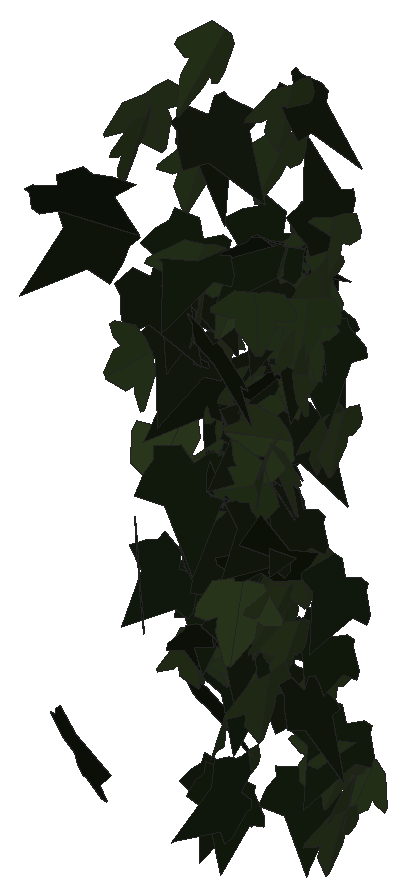
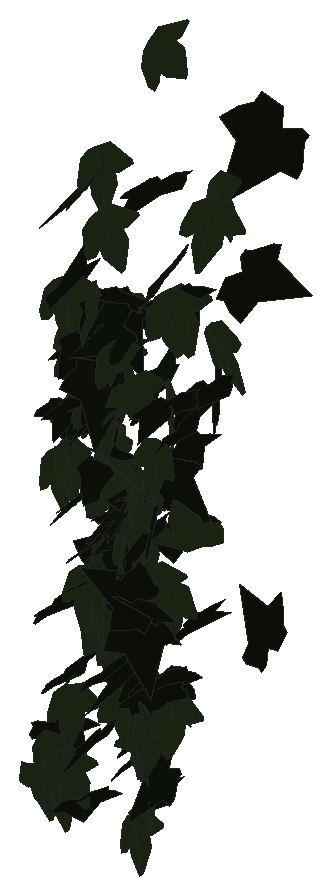
# SketchUp Ruby script. Lengths in inches.
U = 1.inch
M = Sketchup.active_model
def pt(a) = Geom::Point3d.new(a.map { |v| v * U })
def face(e, loops, mat)
  f = e.add_face(loops[0].map { |a| pt(a) })
  loops[1..].each { |l| e.add_face(l.map { |a| pt(a) }).erase! }
  f.material = f.back_material = mat if mat
  f
end
# faces: each face lists its corners as indices into pts; further lists are holes
def faces(e, pts, list, mat = nil) = list.each { |f| face(e, (f[0].is_a?(Array) ? f : [f]).map { |l| l.map { |i| pts[i] } }, mat) }
# xy, xz, yz: faces in a plane at the given z, y or x. An outline is a flat list of corners, or four numbers for a rectangle; further outlines are holes
def ring(l) = l.size == 4 ? [[l[0], l[1]], [l[2], l[1]], [l[2], l[3]], [l[0], l[3]]] : l.each_slice(2).to_a
def flat(e, list, mat, &to3) = list.each { |f| face(e, (f[0].is_a?(Array) ? f : [f]).map { |l| ring(l).map { |u, v| to3.(u, v) } }, mat) }
def xy(e, z, list, mat = nil) = flat(e, list, mat) { |x, y| [x, y, z] }
def xz(e, y, list, mat = nil) = flat(e, list, mat) { |x, z| [x, y, z] }
def yz(e, x, list, mat = nil) = flat(e, list, mat) { |y, z| [x, y, z] }
def lines(e, pts, list) = list.each { |a, b| e.add_line(pt(pts[a]), pt(pts[b])) }
# prism: a flat outline (further loops are holes) pulled along v
def prism(e, loops, v, mat = nil)
  f = face(e, loops, mat); d = Geom::Vector3d.new(v.map { |x| x * U })
  f.pushpull(f.normal.samedirection?(d) ? d.length : -d.length)
end
def box(e, o, s, mat = nil) = prism(e, [[o, [o[0] + s[0], o[1], o[2]], [o[0] + s[0], o[1] + s[1], o[2]], [o[0], o[1] + s[1], o[2]]]], [0, 0, s[2]], mat)
def at(x, y, z, deg = 0) = Geom::Transformation.translation(pt([x, y, z])) * Geom::Transformation.rotation(ORIGIN, Z_AXIS, deg.degrees)
def axes(o, x, y, z) = Geom::Transformation.new([*x, 0, *y, 0, *z, 0, *pt(o).to_a, 1])
def part(name) = M.definitions.add(name)
# library, detail: a bought-in or finely detailed component or shape, given as its bounding box
def library(name, o, s) = part(name).tap { |d| box(d.entities, o, s) }
def detail(e, o, s) = box(e.add_group.entities, o, s)
def put(e, d, t, mat = nil) = e.add_instance(d, t).tap { |i| i.material = mat if mat }
def group(e, t, mat = nil) = e.add_group.tap { |g| g.transformation = t; g.material = mat if mat }.entities
root = M.entities
M.materials.add("efeu1").color = [18, 25, 13]
M.materials.add("efeu2").color = [43, 57, 29]
c1 = part("ivyleaf_10")
p = [[0,0.5,-0.03],[-0.0625,2.02,-0.43],[-0.19,2.01,-0.46],[-0.54,1.05,-0.29],[-0.52,0.625,-0.18],[-0.83,0.76,-0.28],
  [-1.16,0.64,-0.33],[-1.15,0.33,-0.24],[-0.77,-0.39,0.02],[-0.3,-0.51,0.16],[0.04,-0.48,0.23],[-0.02,2.01,-0.4375],
  [-0.06,2.01,-0.43],[0.04,-0.49,0.23],[0.67,-0.49,0.14],[1.38,0.36,-0.2],[1.375,0.51,-0.24],[0.81,0.65,-0.19],
  [0.62,0.59,-0.15],[0.6,1.09,-0.28],[0.5,1.23,-0.31]]
faces(c1.entities,p,[[0,1,2,3,4,5,6,7,8,9,10],[11,12,0,13,14,15,16,17,18,19,20]],"efeu2")
c2 = part("ivyleaf_9")
p = [[1.54,2.16,1.25],[1.36,2.04,1.19],[-0.21,0.99,0.68],[-0.71,1.11,0.82],[-0.85,0.86,0.67],[-0.8,0.17,0.21],
  [-0.9,-0.01,0.1],[-0.67,-0.16,-0.02],[-0.08,-0.08,-0.05],[-0.03,-0.6,-0.4],[0.65,-0.88,-0.66],[0.83,-0.6,-0.49],
  [1.29,-0.42,-0.43],[1.8125,-0.07,-0.26],[1.21,0.44,0.15]]
faces(c2.entities,p,[[0,1,2,3,4,5,6,7,8,9,10,11,12,13,14]],"efeu1")
put(root,c1,axes([530.12,130.77,247.7],[0.59949,0.80925,0.19453],[-0.00458,0.24295,-0.99653],[-0.83229,0.58156,0.14561]))
put(root,c1,axes([530.45,128.96,248.09],[-0.34257,-0.93883,-0.20194],[0.053,0.1956,-0.99924],[0.95884,-0.34624,-0.01692]))
put(root,c2,axes([530.03,129.84,245.78],[0.99528,-0.08963,-0.19402],[-0.19533,-0.00644,-0.99903],[0.08673,1.014,-0.0235]))
put(root,c2,axes([530.17,128.98,261.25],[-0.11198,-1.02799,0.34018],[-0.0593,-0.33566,-1.03385],[1.08119,-0.12488,-0.02147]))
put(root,c1,axes([530.56,128.79,253.32],[-1.05087,0.04613,0.0573],[-0.05724,0.00251,-1.05188],[-0.0462,-1.05242,0]))
put(root,c2,axes([530.78,123.8,266.09],[-0.11934,0.03025,-1.214],[0.21164,-1.20066,-0.05073],[-1.19579,-0.21552,0.11218]))
put(root,c2,axes([530.32,129.95,249.92],[-0.34985,-0.95472,-0.20152],[0.09174,0.18095,-1.01653],[0.97143,-0.36092,0.02343]))
put(root,c2,axes([530.16,130.55,249.63],[-0.1055,-0.93069,-0.43752],[0.16886,0.41817,-0.93025],[1.01444,-0.16639,0.10934]))
put(root,c2,axes([530.61,127.8,251.39],[-0.44294,-0.72773,0.60696],[-0.1684,-0.59888,-0.84094],[0.93254,-0.45381,0.13644]))
put(root,c1,axes([530.68,130.96,248.01],[0.15636,-0.97706,-0.24122],[-0.00188,0.24383,-0.98885],[1.00639,0.15226,0.03563]))
put(root,c2,axes([530.94,129.91,256.45],[0.03772,-0.47428,0.94553],[-0.09107,0.94116,0.47572],[-1.05389,-0.0983,-0.00727]))
put(root,c2,axes([530.18,127.08,262.39],[0.26239,-0.86938,-0.67513],[-0.04832,0.68428,-0.89994],[1.09967,0.23751,0.12155]))
put(root,c1,axes([530.3125,127.43,255.44],[1.01001,0.43056,-0.45145],[0.33211,0.35614,1.08267],[0.52811,-1.04742,0.18255]))
put(root,c1,axes([530.84,129.98,245.01],[0.35064,-0.78367,-0.54081],[-0.16794,0.51638,-0.85715],[0.93724,0.38571,0.04874]))
put(root,c1,axes([530.45,130.86,248.88],[0.85042,-0.50683,0.25032],[0.22614,-0.1094,-0.98977],[0.51807,0.87971,0.02113]))
put(root,c1,axes([530.82,129.52,260.12],[-1.0224,0.29815,0.06081],[-0.05654,0.02331,-1.06497],[-0.29899,-1.02394,-0.00654]))
put(root,c1,axes([530.89,128.79,266.59],[-0.35003,-1.00823,0.27449],[-0.0023,-0.28874,-1.06349],[1.04492,-0.33837,0.08961]))
put(root,c2,axes([531.1,130.24,252.35],[0.13928,0.95863,-0.39167],[-0.04693,-0.38895,-0.96866],[-1.0345,0.14671,-0.00879]))
put(root,c1,axes([530.89,125.92,269.74],[-0.5113,-1.01793,-0.36269],[0.15271,0.32915,-1.13908],[1.06977,-0.53351,-0.01075]))
put(root,c2,axes([530.77,128.34,259.86],[-0.42963,-0.9869,0.13227],[-0.03846,-0.12751,-1.07625],[0.99498,-0.43107,0.01552]))
put(root,c1,axes([530.85,129.02,248.5],[-0.89116,-0.4413,-0.29325],[0.28362,0.08738,-0.9934],[0.44755,-0.93409,0.04561]))
put(root,c1,axes([531.07,130.58,243.11],[-0.05678,-1.01777,-0.0273],[0.00058,0.02731,-1.01936],[1.01814,-0.05677,-0.00094]))
put(root,c2,axes([531.45,128.48,258.46],[0.05872,0.39433,-1.01387],[-0.24983,-0.98332,-0.39692],[-1.05878,0.25389,0.03743]))
put(root,c2,axes([531.35,128.67,249.0625],[0.34784,0.92965,-0.39975],[-0.14348,-0.37312,-0.99259],[-1.00173,0.37626,0.00337]))
put(root,c2,axes([530.73,128.94,262.32],[0.09413,-0.9504,-0.53101],[0.10933,0.53855,-0.94452],[1.08318,0.02823,0.14148]))
put(root,c2,axes([531.2,130.58,253.4],[-0.77358,-0.58488,-0.36776],[0.33791,0.16126,-0.96725],[0.60262,-0.84123,0.07027]))
put(root,c2,axes([530.97,129.97,256.48],[0.41315,-0.87903,-0.41991],[-0.20592,0.367,-0.97089],[0.95216,0.46079,-0.02777]))
put(root,c1,axes([531.28,129.68,257.39],[0.15332,1.02837,-0.21556],[-0.11788,-0.19963,-1.03623],[-1.04409,0.17355,0.08534]))
put(root,c2,axes([531.07,130.69,246.36],[-0.00824,-0.96592,0.32251],[0.05102,-0.32251,-0.96461],[1.01706,0.00835,0.051]))
put(root,c1,axes([531.6,127.72,261.8125],[0.5825,-0.86043,-0.34942],[-0.07373,0.36832,-1.02987],[0.92574,0.57074,0.13784]))
put(root,c2,axes([531.18,129.97,253.33],[0.30859,0.94921,-0.32028],[0.11588,0.29906,0.99797],[0.99506,-0.3292,-0.0169]))
put(root,c1,axes([531.76,124.38,269.77],[0.25662,-1.08207,0.21063],[0.06001,-0.20223,-1.11202],[1.10074,0.26329,0.01152]))
put(root,c1,axes([531.97,128.47,253.37],[-0.41024,-0.92186,0.25569],[-0.07056,-0.24829,-1.0084],[0.95406,-0.41476,0.03536]))
put(root,c2,axes([531.27,128.5,267.68],[0.37366,-1.0709,0.30288],[0.11181,-0.28175,-1.13415],[1.10728,0.38983,0.01232]))
put(root,c2,axes([531.57,127.48,255.68],[-0.32244,-1.11278,-0.29915],[0.12901,0.27382,-1.15764],[1.14505,-0.3442,0.04619]))
put(root,c1,axes([531.8,129.71,258.05],[0.27073,-0.96086,0.35696],[0.19498,-0.31419,-0.9936],[1.00631,0.31938,0.09648]))
put(root,c1,axes([532.11,129.26,255.74],[-0.54822,-0.8563,0.28432],[-0.05627,-0.29959,-1.0108],[0.90051,-0.54003,0.10992]))
put(root,c2,axes([531.93,129.22,251.79],[-0.84528,-0.4313,-0.44212],[0.3754,0.23632,-0.94827],[0.49047,-0.92419,-0.03615]))
put(root,c2,axes([531.79,128.94,243.3125],[-0.20911,-0.94123,0.33342],[-0.04181,-0.3321,-0.96372],[0.99766,-0.2112,0.02949]))
put(root,c1,axes([532.08,129.51,256.86],[0.19886,-1.04332,-0.15253],[0.06117,0.16638,-1.05826],[1.05264,0.18743,0.09031]))
put(root,c1,axes([532.67,123.26,262.1],[0.74777,-0.37964,-0.89561],[-0.74706,0.49937,-0.83542],[0.62301,1.05446,0.07319]))
put(root,c2,axes([531.34,121.66,247.56],[0.15407,-0.39236,1.1611],[0.65177,-0.96482,-0.41251],[1.03793,0.66409,0.08669]))
put(root,c2,axes([531.78,129.83,250.04],[0.47251,-0.61408,-0.7153],[-0.14645,0.74259,-0.73425],[0.93129,0.42834,0.24746]))
put(root,c1,axes([532.35,129.43,255.29],[0.13488,-1.05588,-0.0346],[0.00799,0.0359,-1.06439],[1.05642,0.13454,0.01247]))
put(root,c2,axes([533.11,129.66,258.89],[-0.73823,0.61644,0.46097],[-0.48636,0.12149,-0.94136],[-0.59661,-0.86181,0.19702]))
put(root,c1,axes([532.46,129.04,262.41],[0.53412,0.82489,-0.43726],[-0.3576,-0.28459,-0.97368],[-0.86242,0.62888,0.13292]))
put(root,c1,axes([532.625,129.3125,247.85],[-0.89132,-0.47812,0.19014],[-0.15564,-0.11197,-1.01116],[0.49044,-0.90447,0.02466]))
put(root,c2,axes([532.01,128.99,255.09],[0.38304,-0.99677,0.07006],[0.01635,-0.06877,-1.06779],[0.99909,0.38328,-0.00939]))
put(root,c2,axes([532.13,129.96,257.41],[0.79649,-0.69692,-0.08546],[-0.05915,0.06217,-1.05832],[0.69964,0.79865,0.00781]))
put(root,c1,axes([533,125.9375,264.74],[-0.54976,-0.95739,0.43782],[-0.16961,-0.40692,-1.1028],[1.03899,-0.57301,0.05164]))
put(root,c2,axes([532.94,127.5625,252.09],[-1.03158,0.08408,0.36527],[0.36419,-0.02808,1.035],[0.08863,1.09398,-0.0015]))
put(root,c1,axes([532.8,129.6875,258.23],[0.14132,0.795,-0.70096],[-0.23378,-0.66637,-0.8029],[-1.03379,0.25937,0.08575]))
put(root,c2,axes([532.47,129.91,256.16],[0.07819,-1.05398,0.07923],[0.00586,-0.07901,-1.05688],[1.05694,0.07841,0]))
put(root,c2,axes([532.11,130.0625,255.08],[0.49608,-0.63665,0.68073],[0.40886,-0.54435,-0.80705],[0.83759,0.64278,-0.00923]))
put(root,c2,axes([532.54,128.96,249.57],[-0.06401,-0.9947,0.27218],[0.06025,-0.27584,-0.99392],[1.0295,-0.0457,0.07509]))
put(root,c2,axes([532.56,129.82,256.64],[0.04567,-1.05775,0.09583],[-0.00293,-0.09605,-1.05871],[1.06208,0.04522,-0.00704]))
put(root,c2,axes([532.92,126.19,265.15],[-0.55878,-0.95758,0.09599],[-0.0309,-0.09309,-1.10851],[0.96188,-0.55927,0.02015]))
put(root,c2,axes([532.65,119.27,270.13],[1.09209,0.78995,0.16363],[0.13161,0.09724,-1.34784],[-0.79591,1.09999,0.00164]))
put(root,c2,axes([533.45,129.6,258.75],[-0.24559,0.82548,-0.63707],[-0.04422,-0.66216,-0.84094],[-1.04178,-0.16649,0.18587]))
put(root,c1,axes([533.04,129.45,261.01],[-0.18241,1.05483,0.06532],[-0.04393,0.05866,-1.06996],[-1.05593,-0.18466,0.03323]))
put(root,c2,axes([533.26,129.39,256.63],[-0.57729,-0.69178,0.56472],[-0.18522,-0.56507,-0.88155],[0.87359,-0.57695,0.18628]))
put(root,c2,axes([533.16,130.1,249.36],[-0.22242,-0.96615,0.28906],[0.04103,-0.30443,-0.98595],[1.00763,-0.20087,0.10396]))
put(root,c2,axes([533.01,130.55,246.76],[0.50348,-0.70739,-0.51884],[-0.12405,0.53479,-0.84952],[0.86845,0.4865,0.17944]))
put(root,c1,axes([533.35,129.61,258.51],[-0.8221,-0.61552,-0.30437],[0.31377,0.08559,-1.02058],[0.61078,-0.87245,0.11462]))
put(root,c2,axes([533.75,129.35,262.59],[0.2989,1.03665,-0.02085],[-0.16913,0.02734,-1.0654],[-1.02297,0.29838,0.17005]))
put(root,c1,axes([533.63,128.82,263.39],[-0.17447,-1.06916,0.16961],[-0.004,-0.17116,-1.08305],[1.08252,-0.17295,0.02333]))
put(root,c1,axes([534.35,127.41,256.11],[-0.46385,-0.03418,1.01927],[-0.99443,-0.23328,-0.46037],[0.22627,-1.09529,0.06625]))
put(root,c2,axes([533.33,129.21,255.11],[-0.02323,-1.05348,-0.00984],[0.00051,0.00983,-1.05373],[1.05352,-0.02323,0.00029]))
put(root,c1,axes([533.74,129.14,254.44],[-0.12558,-1.04555,-0.18309],[0.03647,0.18001,-1.05297],[1.06084,-0.12996,0.01453]))
put(root,c1,axes([533.625,127.24,251.7],[1.06375,0.44099,-0.03659],[-0.03726,-0.00567,-1.1515],[-0.44094,1.06436,0.00903]))
put(root,c1,axes([533.88,129.18,252.36],[0.12962,-1.02698,-0.23441],[0.03802,0.24058,-1.03301],[1.05271,0.11776,0.06617]))
put(root,c2,axes([533.04,126.74,261.02],[0.52164,-0.91056,0.61644],[0.37199,-0.49593,-1.04734],[1.03477,0.63731,0.06575]))
put(root,c1,axes([533.9375,128.62,261.89],[-0.87984,0.6414,0.04331],[-0.03262,0.02877,-1.0888],[-0.64203,-0.88044,-0.00403]))
put(root,c2,axes([533.73,126.8,244.75],[-0.11574,-1.00161,0.18712],[0.04156,-0.19281,-1.00635],[1.0181,-0.10599,0.06236]))
put(root,c1,axes([534.83,127.69,257.83],[0.27933,0.01691,-1.05814],[-1.02728,0.26726,-0.26691],[0.25426,1.06125,0.08408]))
put(root,c2,axes([534.64,127.64,264.93],[0.07292,0.8712,-0.65607],[-0.31199,-0.61339,-0.84921],[-1.04503,0.24392,0.20775]))
put(root,c1,axes([534.32,128.58,250.46],[0.01689,-1.05078,-0.14834],[-0.02901,0.14784,-1.05059],[1.06081,0.02077,-0.02636]))
put(root,c2,axes([533.67,125.77,270.21],[0.26945,-0.9044,-0.61716],[0.13905,0.65869,-0.90456],[1.08604,0.14005,0.26893]))
put(root,c2,axes([533.96,130.54,243.32],[-0.26686,-0.97619,-0.13817],[0.18499,0.09102,-1.00037],[0.9684,-0.28639,0.15302]))
put(root,c2,axes([534.71,128.9375,263.74],[0.17806,0.76682,-0.74846],[-0.36329,-0.67059,-0.77346],[-1.00808,0.37711,0.14654]))
put(root,c1,axes([534.78,130.59,244.76],[-0.79743,-0.30381,0.53872],[-0.45971,-0.29688,-0.8479],[0.41375,-0.9154,0.09619]))
put(root,c1,axes([534.48,128.35,251.48],[0.04459,-1.02604,0.41002],[-0.00398,-0.4105,-1.02681],[1.10492,0.03993,-0.02025]))
put(root,c2,axes([534.41,127.97,254.11],[-0.45426,-0.68394,0.65485],[-0.04892,-0.70839,-0.77379],[0.94562,-0.36519,0.27454]))
put(root,c2,axes([534.83,127.91,265.32],[-0.98302,-0.46707,0.08796],[-0.07577,-0.04549,-1.0883],[0.46921,-0.98589,0.00854]))
put(root,c2,axes([534.35,128.4375,262.99],[-0.35633,-1.0252,0.15593],[0.00596,-0.1669,-1.08371],[1.03697,-0.35132,0.05981]))
put(root,c2,axes([533.87,128.16,264.42],[1.02581,0.09267,0.36656],[0.34215,0.22356,-1.014],[-0.16091,1.06615,0.18076]))
put(root,c2,axes([534.01,129.53,261.43],[-0.38886,-0.2086,-0.97796],[0.84515,0.49227,-0.44105],[0.53445,-0.93021,-0.0141]))
put(root,c1,axes([534.72,130.34,247.7],[-0.33241,-0.96187,-0.10175],[0.02363,0.09949,-1.01764],[0.96695,-0.33309,-0.01011]))
put(root,c2,axes([534.26,129.6,260.5],[0.04716,-1.01184,0.34823],[0.01958,-0.34769,-1.01293],[1.0699,0.05096,0.00319]))
put(root,c2,axes([534.42,127.47,252.88],[0.94663,0.32897,0.50604],[-0.47408,-0.17731,1.0021],[0.37356,-1.05865,-0.01059]))
put(root,c1,axes([534.92,127.9375,268.7],[-0.29245,-0.99715,0.41347],[-0.09535,-0.40284,-1.03895],[1.07525,-0.30693,0.02033]))
put(root,c1,axes([534.98,129.07,263.01],[-1.00927,-0.36391,0.1748],[-0.14593,-0.11,-1.07155],[0.37642,-1.01837,0.05328]))
put(root,c1,axes([534.68,127.93,257.02],[-0.89144,0.54624,-0.16724],[0.15477,-0.06743,-1.04523],[-0.5499,-0.90448,-0.02308]))
put(root,c1,axes([534.91,129.06,252.66],[-0.34895,-0.97798,-0.17168],[0.02509,0.17324,-1.03781],[0.99262,-0.34818,-0.03413]))
put(root,c2,axes([534.29,129.66,257.32],[0.44249,-0.89305,-0.33876],[0.04898,0.39407,-0.97488],[0.95388,0.39404,0.2072]))
put(root,c2,axes([534.6,129.28,254.375],[-0.3017,-0.87595,0.49937],[0.07577,-0.53947,-0.90051],[1.00544,-0.22219,0.21771]))
put(root,c1,axes([534.88,128.5,250.21],[0.02965,-0.97597,0.35183],[0.10646,-0.34725,-0.97224],[1.03197,0.06386,0.09019]))
put(root,c1,axes([534.79,128.99,261.4375],[0.2457,1.05115,0.08164],[-0.09951,0.10658,-1.0727],[-1.04961,0.23596,0.12081]))
put(root,c1,axes([535.03,126.9,249.06],[-0.12949,-1.19814,-0.09629],[0.01443,0.09529,-1.20511],[1.20191,-0.13023,0.00409]))
put(root,c2,axes([534.71,130.69,249.02],[-0.21835,-0.93375,0.34678],[0.02703,-0.36044,-0.95351],[0.9957,-0.19498,0.10193]))
put(root,c1,axes([534.8,129.03,265.09],[-0.03865,0.37648,-1.02131],[0.09702,-1.0167,-0.37845],[-1.08416,-0.10441,0.00254]))
put(root,c2,axes([535.73,124.6,246.3],[-1.03988,0.40389,0.05562],[-0.0546,0.01304,-1.11554],[-0.40403,-1.04129,0.00761]))
put(root,c2,axes([534.74,129.79,261.39],[0.09441,-0.96076,-0.45432],[0.05777,0.46007,-0.96092],[1.06119,0.06043,0.09273]))
put(root,c1,axes([535.42,125.99,263.83],[-0.89328,-0.63308,0.04333],[-0.0364,-0.02357,-1.09487],[0.63351,-0.89402,-0.00181]))
put(root,c1,axes([534.9,127.18,257.3],[-0.17418,-0.2576,-1.08193],[0.30362,-1.06454,0.20458],[-1.06993,-0.26015,0.23419]))
put(root,c2,axes([535.17,129.66,260.98],[-0.42013,-0.8611,-0.47341],[0.2533,0.40257,-0.95703],[0.94945,-0.48843,0.04584]))
put(root,c2,axes([535.56,130.3125,246.2],[-0.70532,-0.72939,-0.04705],[0.03409,0.03248,-1.01463],[0.73011,-0.70614,0.00193]))
put(root,c1,axes([535.71,127.23,271.12],[-0.24424,-1.11085,0.02732],[-0.00521,-0.02683,-1.13738],[1.11117,-0.2443,0.00067]))
put(root,c1,axes([535.79,130.26,245.27],[-0.24256,-0.89885,0.38975],[-0.04245,-0.3915,-0.9293],[0.97879,-0.23973,0.05628]))
put(root,c1,axes([535.78,131.26,244.19],[0.92728,-0.20646,-0.31299],[-0.28083,0.1708,-0.94466],[0.24844,0.96365,0.10038]))
put(root,c1,axes([535.67,123.42,274.65],[-0.08369,-0.86997,0.8758],[0.19441,-0.87614,-0.85174],[1.21905,0.08,0.19595]))
put(root,c1,axes([535.7,127.85,262.04],[-0.59746,-0.85008,-0.28649],[0.24227,0.17852,-1.03494],[0.86372,-0.6381,0.09212]))
put(root,c1,axes([535.86,129.11,258.18],[0.11835,-1.06133,-0.04109],[-0.02322,0.03875,-1.06774],[1.06187,0.11913,-0.01877]))
put(root,c1,axes([535.84,128.66,263.85],[-0.15123,-0.99555,-0.3844],[0.06378,0.37911,-1.00696],[1.06528,-0.16403,0.00572]))
put(root,c1,axes([535.77,127.8125,262.05],[-0.08791,-0.92592,-0.55194],[0.15596,0.53702,-0.92574],[1.06661,-0.15484,0.08987]))
put(root,c1,axes([535.86,130.21,244.08],[0.28328,-0.95506,-0.17778],[-0.03529,0.17494,-0.99606],[0.97082,0.28504,0.01566]))
put(root,c1,axes([535.89,129.68,243.04],[-0.04682,-1.03351,0.08589],[-0.01391,-0.08534,-1.03452],[1.03698,-0.04781,-0.01]))
put(root,c2,axes([536.08,128.96,265.61],[-0.38299,-0.85783,0.56778],[0.22924,0.51945,0.93945],[-1.00285,0.44635,-0.00209]))
put(root,c2,axes([535.63,130.21,251.73],[-0.30066,-0.91202,0.39949],[-0.03146,-0.40839,-0.95603],[0.99517,-0.28845,0.09046]))
put(root,c1,axes([536.13,127.39,260.79],[-0.19426,0.49194,0.97774],[-0.58552,0.79228,-0.51496],[-0.92474,-0.60499,0.12066]))
put(root,c1,axes([535.98,129.54,258.03],[-0.17283,-1.05243,0.04669],[0.02758,-0.05181,-1.06593],[1.05311,-0.17136,0.03558]))
put(root,c2,axes([535.375,128.13,270.73],[0.78818,-0.69825,-0.40956],[-0.11206,0.47202,-1.02038],[0.80171,0.75244,0.26003]))
put(root,c1,axes([536.15,128.9,265.625],[-0.47304,-0.98362,0.12394],[-0.00913,-0.13299,-1.09035],[0.99135,-0.47057,0.04909]))
put(root,c2,axes([535.5,128.44,248.23],[0.5033,-0.9154,-0.19086],[-0.04316,0.19378,-1.0432],[0.93409,0.50218,0.05464]))
put(root,c2,axes([535.56,119.72,256.16],[-0.01789,0.07483,1.28295],[0.14848,-1.27436,0.0764],[1.27652,0.14927,0.00909]))
put(root,c1,axes([536.24,127.58,263.18],[-0.63223,-0.86868,0.12919],[-0.0518,-0.12202,-1.07398],[0.8767,-0.63365,0.0297]))
